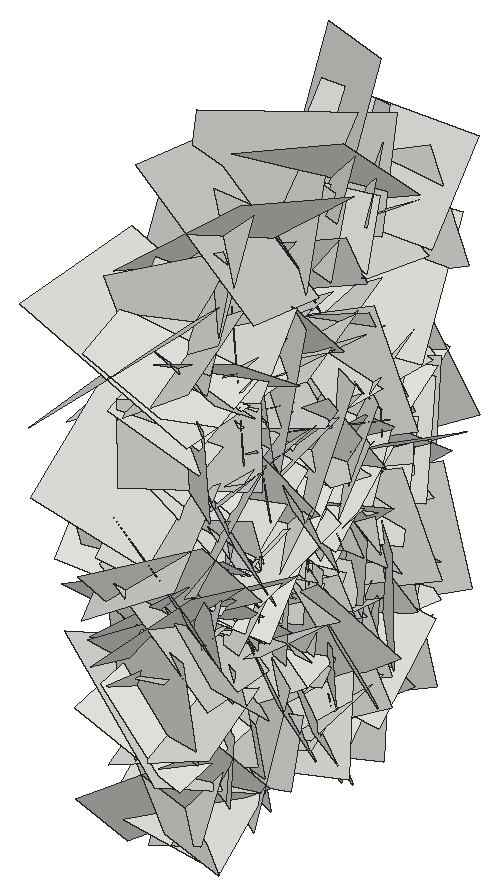
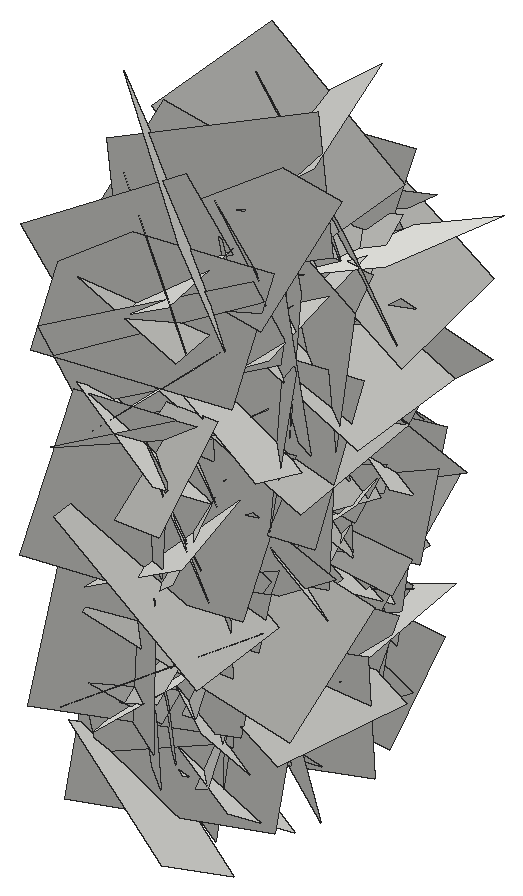
# SketchUp Ruby script. Lengths in inches.
U = 1.inch
M = Sketchup.active_model
def pt(a) = Geom::Point3d.new(a.map { |v| v * U })
def face(e, loops, mat)
  f = e.add_face(loops[0].map { |a| pt(a) })
  loops[1..].each { |l| e.add_face(l.map { |a| pt(a) }).erase! }
  f.material = f.back_material = mat if mat
  f
end
# faces: each face lists its corners as indices into pts; further lists are holes
def faces(e, pts, list, mat = nil) = list.each { |f| face(e, (f[0].is_a?(Array) ? f : [f]).map { |l| l.map { |i| pts[i] } }, mat) }
# xy, xz, yz: faces in a plane at the given z, y or x. An outline is a flat list of corners, or four numbers for a rectangle; further outlines are holes
def ring(l) = l.size == 4 ? [[l[0], l[1]], [l[2], l[1]], [l[2], l[3]], [l[0], l[3]]] : l.each_slice(2).to_a
def flat(e, list, mat, &to3) = list.each { |f| face(e, (f[0].is_a?(Array) ? f : [f]).map { |l| ring(l).map { |u, v| to3.(u, v) } }, mat) }
def xy(e, z, list, mat = nil) = flat(e, list, mat) { |x, y| [x, y, z] }
def xz(e, y, list, mat = nil) = flat(e, list, mat) { |x, z| [x, y, z] }
def yz(e, x, list, mat = nil) = flat(e, list, mat) { |y, z| [x, y, z] }
def lines(e, pts, list) = list.each { |a, b| e.add_line(pt(pts[a]), pt(pts[b])) }
# prism: a flat outline (further loops are holes) pulled along v
def prism(e, loops, v, mat = nil)
  f = face(e, loops, mat); d = Geom::Vector3d.new(v.map { |x| x * U })
  f.pushpull(f.normal.samedirection?(d) ? d.length : -d.length)
end
def box(e, o, s, mat = nil) = prism(e, [[o, [o[0] + s[0], o[1], o[2]], [o[0] + s[0], o[1] + s[1], o[2]], [o[0], o[1] + s[1], o[2]]]], [0, 0, s[2]], mat)
def at(x, y, z, deg = 0) = Geom::Transformation.translation(pt([x, y, z])) * Geom::Transformation.rotation(ORIGIN, Z_AXIS, deg.degrees)
def axes(o, x, y, z) = Geom::Transformation.new([*x, 0, *y, 0, *z, 0, *pt(o).to_a, 1])
def part(name) = M.definitions.add(name)
# library, detail: a bought-in or finely detailed component or shape, given as its bounding box
def library(name, o, s) = part(name).tap { |d| box(d.entities, o, s) }
def detail(e, o, s) = box(e.add_group.entities, o, s)
def put(e, d, t, mat = nil) = e.add_instance(d, t).tap { |i| i.material = mat if mat }
def group(e, t, mat = nil) = e.add_group.tap { |g| g.transformation = t; g.material = mat if mat }.entities
root = M.entities
c1 = part("Component\#6")
p = [[0.01,0,0],[0,3.24,4.54],[4.32,3.24,4.54],[4.33,0,0]]
faces(c1.entities,p,[[0,1,2,3]])
put(root,c1,axes([18.5,148.21,18.05],[-0.18781,1.38239,0.05917],[-0.11095,0.04609,-1.39025],[-1.46247,-0.18102,0.09787]))
put(root,c1,axes([18.5,151.36,16.73],[-0.05564,-1.33407,-0.12972],[-0.26745,-0.11766,1.31218],[-1.39538,0.07575,-0.24633]))
put(root,c1,axes([18.5,153.54,10.59],[-0.17173,1.22834,-0.55665],[-0.01226,-0.5619,-1.23655],[-1.42944,-0.14275,0.07748]))
put(root,c1,axes([18.5,150.02,13.53],[-0.11354,-0.10924,1.28227],[-0.18202,1.27641,0.09439],[-1.35193,-0.16268,-0.1204]))
put(root,c1,axes([18.5,150.46,17.01],[-0.04698,1.34267,-0.16756],[-0.13374,-0.17102,-1.33703],[-1.42802,-0.02815,0.13073]))
put(root,c1,axes([18.5,146.56,18.67],[-0.08115,0.67304,1.19325],[-0.03541,1.19384,-0.67552],[-1.45175,-0.06674,-0.05023]))
put(root,c1,axes([18.5,155.15,17.37],[-0.02517,0.60882,-1.16754],[-0.2041,-1.15679,-0.59929],[-1.38075,0.1599,0.10987]))
put(root,c1,axes([18.5,149.47,1.18],[-0.22795,-1.08393,0.44752],[-0.03192,0.45993,1.09954],[-1.24263,0.18702,-0.11034]))
put(root,c1,axes([18.5,145.22,20.96],[-0.20751,1.35949,-0.09859],[0.20583,-0.07077,-1.36145],[-1.43011,-0.20745,-0.18164]))
put(root,c1,axes([18.5,151.77,16.16],[-0.14743,1.12249,0.38129],[-0.0578,0.37744,-1.13105],[-1.25528,-0.14922,0.00729]))
put(root,c1,axes([18.5,155.16,12.125],[-0.20792,1.23942,0.0793],[0.14973,0.10203,-1.24521],[-1.30793,-0.18535,-0.15516]))
put(root,c1,axes([18.5,149.82,11.51],[-0.16938,-0.10345,1.35904],[0.25816,1.34416,0.13095],[-1.4215,0.25644,-0.13816]))
put(root,c1,axes([18.5,149.27,6.59],[0.15688,1.33929,-0.00269],[-0.18956,0.01708,-1.33541],[-1.40693,0.14704,0.17962]))
put(root,c1,axes([18.5,157.09,9.16],[-0.26081,-0.66319,-0.77037],[-0.09697,-0.77495,0.69635],[-1.07312,0.23121,0.12431]))
put(root,c1,axes([18.5,153.21,11.43],[0.14123,-0.96535,-0.93141],[-0.15435,-0.94087,0.95433],[-1.41351,0.00629,-0.19727]))
put(root,c1,axes([18.5,154.4,5.48],[0.14525,-0.2612,-1.20099],[-0.27145,-1.18798,0.22915],[-1.27422,0.2233,-0.18571]))
put(root,c1,axes([18.5,153.41,21.56],[-0.04666,0.60871,1.19242],[0.17987,1.18598,-0.59916],[-1.40769,0.13136,-0.11609]))
put(root,c1,axes([18.5,152.41,8.09],[0.02535,-1.06677,0.60381],[-0.0625,0.60222,1.06631],[-1.29785,-0.04984,-0.03955]))
put(root,c1,axes([18.5,151.84,12.71],[-0.09641,-0.969,-0.91768],[0.24854,-0.9171,0.94515],[-1.39265,-0.09659,0.2322]))
put(root,c1,axes([18.5,148.37,14.37],[-0.13394,0.02599,1.3483],[0.3112,1.32226,0.00203],[-1.39518,0.29244,-0.12899]))
put(root,c1,axes([18.5,148.8125,12.02],[-0.02959,0.36254,-1.01381],[-0.21176,-0.99828,-0.35148],[-1.12146,0.17893,0.09312]))
put(root,c1,axes([18.5,153.72,24.55],[0.10736,0.8301,-0.78481],[-0.26067,-0.75358,-0.8288],[-1.18252,0.24148,0.11144]))
put(root,c1,axes([18.5,144.59,11.1],[-0.20686,0.83944,0.54314],[-0.00436,0.55271,-0.85571],[-1.05982,-0.16612,-0.10249]))
put(root,c1,axes([18.5,150.33,13.2],[0.24126,0.02501,1.36725],[-0.05252,1.3853,-0.01709],[-1.44858,-0.04606,0.22834]))
put(root,c1,axes([18.5,153.16,13.74],[-0.07693,-1.07175,0.44962],[0.07215,0.4458,1.07364],[-1.22986,0.09319,0.03486]))
put(root,c1,axes([14.53,155.94,6.59],[-0.14653,0.65267,0.04592],[-0.0729,0.03218,-0.6644],[0.6897,0.14207,-0.06047]))
put(root,c1,axes([18.5,147.25,11.15],[-0.01251,0.83252,-0.66438],[-0.16644,-0.65852,-0.82239],[-1.1167,0.08883,0.13002]))
put(root,c1,axes([18.5,157.5,5.99],[-0.02733,0.34478,-1.12821],[0.04378,-1.12752,-0.34552],[-1.24973,-0.04704,0.01257]))
put(root,c1,axes([18.5,159.05,4.5],[-0.22831,-0.97739,-0.02602],[0.01319,-0.02938,1.00067],[-1.03632,0.21495,0.01847]))
put(root,c1,axes([18.5,156.09,10.89],[-0.02844,-1.01096,-0.23497],[-0.17327,-0.228,0.99963],[-1.08645,0.06282,-0.15327]))
put(root,c1,axes([18.5,158.38,15.93],[0.03304,0.59909,-1.16183],[0.1621,-1.15585,-0.5919],[-1.37611,-0.12177,-0.09762]))
put(root,c1,axes([18.5,147.43,1.76],[-0.0449,0.15818,1.07958],[-0.0304,1.07985,-0.15935],[-1.15617,-0.03454,-0.03773]))
put(root,c1,axes([18.5,156.6875,24.44],[-0.16473,0.01802,-1.18121],[0.23771,-1.16927,-0.04735],[-1.22945,-0.22849,0.14911]))
put(root,c1,axes([14.53,148.65,3.04],[-0.12439,-0.47488,0.46679],[-0.05284,0.47892,0.47469],[0.70386,-0.04797,0.11813]))
put(root,c1,axes([14.53,150.18,6.375],[-0.17639,-0.58204,-0.33942],[0.00316,-0.35025,0.59915],[0.71419,-0.1422,-0.08648]))
put(root,c1,axes([18.5,151.75,19.45],[-0.16935,0.44212,0.83371],[-0.05466,0.84022,-0.45546],[-0.99881,-0.12095,-0.11643]))
put(root,c1,axes([18.5,152.08,1.74],[-0.04493,0.85391,0.54577],[-0.09586,0.54089,-0.85328],[-1.06994,-0.08432,0.05353]))
put(root,c1,axes([18.5,158.83,13.98],[-0.00743,-1.2386,0.03478],[0.17851,0.0335,1.22715],[-1.30124,0.01167,0.16814]))
put(root,c1,axes([18.5,148.93,-0.125],[0.17085,0.2332,1.25619],[0.02467,1.2654,-0.2379],[-1.35409,0.05247,0.15416]))
put(root,c1,axes([18.5,148.09,7.11],[0.15706,0.67864,1.02073],[-0.03183,1.02986,-0.68036],[-1.29889,0.05683,0.1401]))
put(root,c1,axes([18.5,145.87,3.84],[-0.08046,-0.07863,0.91675],[-0.19442,0.90269,0.06223],[-0.95574,-0.17701,-0.08983]))
put(root,c1,axes([18.5,155.4,17.52],[0.19723,0.3027,-1.19403],[-0.0763,-1.20284,-0.31615],[-1.30348,0.11621,-0.16216]))
put(root,c1,axes([18.5,148.31,17.26],[-0.09379,0.98835,0.28145],[0.01751,0.28383,-0.99149],[-1.08916,-0.08054,-0.04018]))
put(root,c1,axes([18.5,151.01,19.39],[-0.01021,0.65154,-0.69294],[-0.23408,-0.67557,-0.63214],[-0.98066,0.15447,0.1581]))
put(root,c1,axes([18.5,157.43,12.97],[0.1074,-0.05602,-1.35571],[0.22854,-1.34155,0.07155],[-1.42001,-0.22014,-0.09102]))
put(root,c1,axes([14.53,152.72,13.34],[-0.14332,-0.62648,-0.12325],[0.10799,-0.14554,0.62801],[0.66813,-0.11086,-0.12794]))
put(root,c1,axes([18.5,154.9,1.8],[-0.03269,0.90387,0.50014],[-0.00572,0.50021,-0.90434],[-1.09498,-0.0296,-0.01021]))
put(root,c1,axes([14.53,149.02,5.32],[-0.19432,-0.67994,0.40742],[-0.04988,0.42677,0.69106],[0.83874,-0.13215,0.13549]))
put(root,c1,axes([18.5,160.22,19.0625],[0.13961,-0.68099,-1.03193],[0.07146,-1.03227,0.68982],[-1.30861,-0.12902,-0.07242]))
put(root,c1,axes([18.5,157.74,11.21],[-0.0595,-0.6331,0.72554],[-0.06262,0.72766,0.63038],[-1.01877,-0.00775,-0.08112]))
put(root,c1,axes([14.53,146,16.15],[-0.10062,0.63244,0.10884],[0.07256,0.11937,-0.63396],[0.67636,0.08128,0.0842]))
put(root,c1,axes([14.53,147.25,18.09],[-0.11506,-0.20062,0.68841],[-0.02156,0.69683,0.19986],[0.75976,-0.01061,0.10993]))
put(root,c1,axes([14.53,155.37,8.05],[-0.03179,-0.04018,0.69029],[-0.07893,0.6871,0.03676],[0.72868,0.07267,0.03409]))
put(root,c1,axes([14.53,151.91,13.09],[-0.06029,-0.61389,0.14039],[0.0496,0.13645,0.61563],[0.66568,-0.06576,-0.03315]))
put(root,c1,axes([18.5,153.47,7.93],[0.25077,0.36385,-1.26635],[0.08689,-1.28818,-0.35481],[-1.39394,-0.01484,-0.24993]))
put(root,c1,axes([18.5,158.45,22.43],[0.19892,0.24365,-1.12098],[-0.08242,-1.13056,-0.25875],[-1.21318,0.11676,-0.16622]))
put(root,c1,axes([14.53,151.13,9.12],[-0.15296,0.67587,0.31221],[0.03502,0.32352,-0.68509],[0.78839,0.11676,0.09101]))
put(root,c1,axes([18.5,148.76,4.0625],[-0.10183,-0.75916,-0.2873],[-0.20096,-0.26032,0.75126],[-0.83661,0.15493,-0.14549]))
put(root,c1,axes([18.5,155.05,20.66],[-0.11898,0.43702,0.87755],[0.10329,0.88388,-0.42771],[-1.03402,0.038,-0.1437]))
put(root,c1,axes([18.5,154.79,8.7],[0.06507,0.61236,-0.89404],[0.03144,-0.89608,-0.61173],[-1.14823,0.01016,-0.06741]))
put(root,c1,axes([14.53,151.99,2.12],[-0.1775,0.68354,0.35821],[0.06031,0.37649,-0.69181],[0.81579,0.12089,0.12909]))
put(root,c1,axes([14.53,151.79,4.27],[-0.00282,-0.67031,0.14172],[-0.04158,0.14164,0.66918],[0.72504,0.00552,0.03892]))
put(root,c1,axes([14.53,147.62,1.41],[-0.08717,-0.06025,0.7019],[0.04865,0.70471,0.06586],[0.74517,-0.05306,0.07781]))
put(root,c1,axes([14.53,156.87,7.65],[0.00449,0.50233,-0.39291],[0.02578,-0.39276,-0.50188],[0.67552,0.01165,0.02176]))
put(root,c1,axes([14.53,153.92,20.8125],[0.01755,0.277,-0.54123],[0.05617,-0.54003,-0.27476],[0.64202,0.03967,0.03883]))
put(root,c1,axes([18.5,152.6,3.91],[-0.02426,0.68313,0.69515],[0.0107,0.69547,-0.68312],[-1.03305,-0.00884,-0.0234]))
put(root,c1,axes([14.53,147.13,6.96],[-0.04816,-0.19283,0.63159],[0.07038,0.62854,0.19668],[0.69645,-0.07685,0.0238]))
put(root,c1,axes([18.5,158.68,8.63],[0.07829,-0.94373,0.27717],[-0.10215,0.26967,0.94388],[-1.03759,-0.09775,-0.07202]))
put(root,c1,axes([18.5,152.91,14.99],[0.05042,0.65822,-0.8803],[0.11398,-0.87969,-0.65195],[-1.15954,-0.05785,-0.10236]))
put(root,c1,axes([18.5,159.16,9.85],[0.13765,0.1916,-1.18129],[0.14512,-1.1828,-0.17679],[-1.2602,-0.11528,-0.14939]))
put(root,c1,axes([18.5,157.06,14.03],[0.04606,-0.47436,-0.98882],[0.12961,-0.98133,0.47614],[-1.15527,-0.12901,0.01399]))
put(root,c1,axes([18.5,149.64,15.49],[0.05397,-0.71515,0.49033],[-0.26351,0.45852,0.69456],[-0.88054,-0.18105,-0.1778]))
put(root,c1,axes([14.53,148.39,13.69],[0.056,0.56116,0.2115],[0.06403,0.20626,-0.56234],[0.63244,-0.07057,0.03821]))
put(root,c1,axes([18.5,147.71,9.53],[0.0202,0.73421,-0.62443],[-0.01239,-0.62433,-0.73445],[-1.02159,0.02209,-0.00344]))
put(root,c1,axes([14.53,146.72,8.375],[0.05548,0.31048,0.67068],[-0.12303,0.66747,-0.29994],[0.77368,0.08387,-0.09579]))
put(root,c1,axes([18.5,152.28,1.18],[0.22482,-0.75958,0.923],[0.06114,0.94282,0.76264],[-1.2656,-0.08938,0.2008]))
put(root,c1,axes([18.5,154.73,4.99],[0.23466,-0.21907,1.02966],[-0.17179,1.03255,0.25453],[-1.10257,-0.20751,0.17949]))
put(root,c1,axes([14.53,148.44,10.1],[0.02371,0.59128,0.15103],[0.13632,0.14317,-0.57956],[0.63236,-0.05303,0.11928]))
put(root,c1,axes([14.53,154.81,5.31],[0.03271,-0.68931,-0.29186],[-0.0897,-0.29345,0.68411],[0.78838,-0.00479,0.08995]))
put(root,c1,axes([14.53,155.07,5.6],[-0.26442,-0.95782,0.42161],[-0.12666,0.45666,0.96674],[1.10204,-0.17733,0.21227]))
put(root,c1,axes([18.5,146.38,17.95],[-0.09245,0.38694,0.78979],[0.04684,0.79459,-0.38441],[-0.93107,0.00155,-0.09776]))
put(root,c1,axes([14.53,155.43,2.74],[0.05213,0.12024,0.7107],[-0.06472,0.71048,-0.11598],[0.7613,0.05216,-0.05853]))
put(root,c1,axes([18.5,149.03,14.67],[0.12882,0.64149,-0.81464],[-0.00451,-0.8199,-0.64626],[-1.09909,0.07855,-0.09282]))
put(root,c1,axes([14.53,145.53,10.42],[-0.22479,1.04725,-0.16356],[-0.16331,-0.19548,-1.05191],[1.11161,0.18306,-0.18761]))
put(root,c1,axes([18.5,147.21,13.43],[0.06341,1.09172,0.23851],[0.19798,0.22572,-1.08003],[-1.16785,0.09755,-0.17015]))
put(root,c1,axes([14.53,146.09,12.1875],[-0.18427,0.52878,-0.65011],[0.11203,-0.64482,-0.55274],[0.8812,0.19255,-0.06567]))
put(root,c1,axes([18.5,151.57,3.27],[-0.14157,0.02397,-0.74069],[-0.04702,-0.75154,-0.01632],[-0.78414,0.04073,0.1347]))
put(root,c1,axes([14.53,154.48,3.89],[0.11783,0.23417,0.69133],[-0.11259,0.69704,-0.21902],[0.76547,0.06648,-0.13863]))
put(root,c1,axes([14.53,152.53,7.1875],[0.08757,-0.64703,0.3684],[-0.09594,0.35919,0.65114],[0.78338,0.11632,0.03856]))
put(root,c1,axes([18.5,153.68,-0.24],[-0.08313,-0.05331,0.78078],[-0.05564,0.78328,0.04821],[-0.82769,-0.0473,-0.08166]))
put(root,c1,axes([14.53,155.23,10.47],[-0.04155,0.12694,-0.87349],[-0.11983,-0.86787,-0.12105],[0.92792,-0.10639,-0.05475]))
put(root,c1,axes([18.5,154.93,13.48],[0.13332,0.92748,-0.67904],[0.1887,-0.69057,-0.91025],[-1.20375,-0.00553,-0.2179]))
put(root,c1,axes([18.5,152.46,19.1],[0.24316,-1.11668,0.32256],[0.08367,0.34299,1.13127],[-1.22923,-0.19755,0.14081]))
put(root,c1,axes([18.5,149.625,17.57],[-0.05592,-0.7816,-0.40589],[0.0657,-0.4089,0.77935],[-0.93124,0.01809,0.07936]))
put(root,c1,axes([14.53,153.02,6.56],[0.04835,0.51462,-0.41299],[0.10228,-0.41473,-0.50612],[0.69191,0.02534,0.10368]))
put(root,c1,axes([14.53,155.74,21.65],[-0.00825,-0.17983,-0.66547],[0.14401,-0.65286,0.17483],[0.71636,0.12918,-0.04281]))
put(root,c1,axes([18.5,147.06,-0.97],[-0.01135,-0.66277,0.66685],[0.09721,0.66298,0.66039],[-0.99185,0.07256,0.05709]))
put(root,c1,axes([14.53,154.86,6.54],[-0.11481,0.21277,-0.79232],[0.09254,-0.79167,-0.22453],[0.86468,0.11298,-0.08117]))
put(root,c1,axes([18.5,155.95,10.68],[-0.04823,-0.00518,0.84226],[0.02844,0.84305,0.00663],[-0.89236,0.02715,-0.04531]))
put(root,c1,axes([18.5,146.53,12.92],[-0.03124,-0.05121,0.8385],[0.00373,0.839,0.05136],[-0.89046,0.00531,-0.0292]))
put(root,c1,axes([18.5,152.8,10.75],[0.04843,-0.82009,-0.82841],[0.32646,-0.79109,0.80013],[-1.19171,-0.25004,0.18553]))
put(root,c1,axes([14.53,155.82,10.86],[-0.10869,-0.77244,0.23734],[0.13092,0.22145,0.77409],[0.8465,-0.13343,-0.08925]))
put(root,c1,axes([14.53,156.49,11.61],[-0.16435,-0.92659,-0.48849],[-0.14398,-0.47186,0.93815],[1.10094,-0.20004,0.04977]))
put(root,c1,axes([18.5,153.88,7.81],[-0.12498,-0.19712,-0.75186],[0.05107,-0.76085,0.19192],[-0.82232,-0.01729,0.12619]))
put(root,c1,axes([14.53,154.72,7.86],[0.01434,-0.12328,-0.7123],[0.10241,-0.70572,0.12398],[0.75939,0.0975,-0.00327]))
put(root,c1,axes([18.5,155.22,14.18],[0.0107,0.67836,0.43703],[-0.08223,0.43585,-0.67474],[-0.8514,-0.03357,0.07066]))
put(root,c1,axes([14.53,152.55,8.85],[-0.17208,0.39932,0.93109],[-0.08126,0.93542,-0.41455],[1.07081,0.13515,0.11817]))
put(root,c1,axes([18.5,155.14,21.07],[0.01676,0.7943,-0.14622],[-0.08914,-0.14383,-0.79043],[-0.85145,0.03069,0.07988]))
put(root,c1,axes([14.53,158.76,13.54],[-0.17018,-0.33172,-0.9968],[-0.1229,-0.99662,0.35033],[1.10678,-0.16167,-0.11436]))
put(root,c1,axes([18.5,151.77,10.3],[-0.00621,-0.04081,-0.81439],[-0.02737,-0.814,0.04098],[-0.86391,0.02608,0.00455]))
put(root,c1,axes([18.5,149.67,1.32],[-0.10197,-0.47157,-0.58691],[0.00963,-0.59236,0.47447],[-0.798,0.05311,0.08072]))
put(root,c1,axes([14.53,154.27,5.56],[-0.10843,0.64197,-0.78685],[-0.13439,-0.79271,-0.63027],[1.06801,-0.03458,-0.15919]))
put(root,c1,axes([18.5,154.27,5.56],[0.10843,0.64197,-0.78685],[0.13439,-0.79271,-0.63027],[-1.06801,-0.03458,-0.15919]))
put(root,c1,axes([14.53,149.67,1.32],[0.10197,-0.47157,-0.58691],[-0.00963,-0.59236,0.47447],[0.798,0.05311,0.08072]))
put(root,c1,axes([14.53,151.77,10.3],[0.00621,-0.04081,-0.81439],[0.02737,-0.814,0.04098],[0.86391,0.02608,0.00455]))
put(root,c1,axes([18.5,158.76,13.54],[0.17018,-0.33172,-0.9968],[0.1229,-0.99662,0.35033],[-1.10678,-0.16167,-0.11436]))
put(root,c1,axes([14.53,155.14,21.07],[-0.01676,0.7943,-0.14622],[0.08914,-0.14383,-0.79043],[0.85145,0.03069,0.07988]))
put(root,c1,axes([18.5,152.55,8.85],[0.17208,0.39932,0.93109],[0.08126,0.93542,-0.41455],[-1.07081,0.13515,0.11817]))
put(root,c1,axes([14.53,155.22,14.18],[-0.0107,0.67836,0.43703],[0.08223,0.43585,-0.67474],[0.8514,-0.03357,0.07066]))
put(root,c1,axes([18.5,154.72,7.86],[-0.01434,-0.12328,-0.7123],[-0.10241,-0.70572,0.12398],[-0.75939,0.0975,-0.00327]))
put(root,c1,axes([14.53,153.88,7.81],[0.12498,-0.19712,-0.75186],[-0.05107,-0.76085,0.19192],[0.82232,-0.01729,0.12619]))
put(root,c1,axes([18.5,156.49,11.61],[0.16435,-0.92659,-0.48849],[0.14398,-0.47186,0.93815],[-1.10094,-0.20004,0.04977]))
put(root,c1,axes([18.5,155.82,10.86],[0.10869,-0.77244,0.23734],[-0.13092,0.22145,0.77409],[-0.8465,-0.13343,-0.08925]))
put(root,c1,axes([14.53,152.8,10.75],[-0.04843,-0.82009,-0.82841],[-0.32646,-0.79109,0.80013],[1.19171,-0.25004,0.18553]))
put(root,c1,axes([14.53,146.53,12.92],[0.03124,-0.05121,0.8385],[-0.00373,0.839,0.05136],[0.89046,0.00531,-0.0292]))
put(root,c1,axes([14.53,155.95,10.68],[0.04823,-0.00518,0.84226],[-0.02844,0.84305,0.00663],[0.89236,0.02715,-0.04531]))
put(root,c1,axes([18.5,154.86,6.54],[0.11481,0.21277,-0.79232],[-0.09254,-0.79167,-0.22453],[-0.86468,0.11298,-0.08117]))
put(root,c1,axes([14.53,147.06,-0.97],[0.01135,-0.66277,0.66685],[-0.09721,0.66298,0.66039],[0.99185,0.07256,0.05709]))
put(root,c1,axes([18.5,155.74,21.65],[0.00825,-0.17983,-0.66547],[-0.14401,-0.65286,0.17483],[-0.71636,0.12918,-0.04281]))
put(root,c1,axes([18.5,153.02,6.56],[-0.04835,0.51462,-0.41299],[-0.10228,-0.41473,-0.50612],[-0.69191,0.02534,0.10368]))
put(root,c1,axes([14.53,149.625,17.57],[0.05592,-0.7816,-0.40589],[-0.0657,-0.4089,0.77935],[0.93124,0.01809,0.07936]))
put(root,c1,axes([14.53,152.46,19.1],[-0.24316,-1.11668,0.32256],[-0.08367,0.34299,1.13127],[1.22923,-0.19755,0.14081]))
put(root,c1,axes([14.53,154.93,13.48],[-0.13332,0.92748,-0.67904],[-0.1887,-0.69057,-0.91025],[1.20375,-0.00553,-0.2179]))
put(root,c1,axes([18.5,155.23,10.47],[0.04155,0.12694,-0.87349],[0.11983,-0.86787,-0.12105],[-0.92792,-0.10639,-0.05475]))
put(root,c1,axes([14.53,153.68,-0.24],[0.08313,-0.05331,0.78078],[0.05564,0.78328,0.04821],[0.82769,-0.0473,-0.08166]))
put(root,c1,axes([18.5,152.53,7.1875],[-0.08757,-0.64703,0.3684],[0.09594,0.35919,0.65114],[-0.78338,0.11632,0.03856]))
put(root,c1,axes([18.5,154.48,3.89],[-0.11783,0.23417,0.69133],[0.11259,0.69704,-0.21902],[-0.76547,0.06648,-0.13863]))
put(root,c1,axes([14.53,151.57,3.27],[0.14157,0.02397,-0.74069],[0.04702,-0.75154,-0.01632],[0.78414,0.04073,0.1347]))
put(root,c1,axes([18.5,146.09,12.1875],[0.18427,0.52878,-0.65011],[-0.11203,-0.64482,-0.55274],[-0.8812,0.19255,-0.06567]))
put(root,c1,axes([14.53,147.21,13.43],[-0.06341,1.09172,0.23851],[-0.19798,0.22572,-1.08003],[1.16785,0.09755,-0.17015]))
put(root,c1,axes([18.5,145.53,10.42],[0.22479,1.04725,-0.16356],[0.16331,-0.19548,-1.05191],[-1.11161,0.18306,-0.18761]))
put(root,c1,axes([14.53,149.03,14.67],[-0.12882,0.64149,-0.81464],[0.00451,-0.8199,-0.64626],[1.09909,0.07855,-0.09282]))
put(root,c1,axes([18.5,155.43,2.74],[-0.05213,0.12024,0.7107],[0.06472,0.71048,-0.11598],[-0.7613,0.05216,-0.05853]))
put(root,c1,axes([14.53,146.38,17.95],[0.09245,0.38694,0.78979],[-0.04684,0.79459,-0.38441],[0.93107,0.00155,-0.09776]))
put(root,c1,axes([18.5,155.07,5.6],[0.26442,-0.95782,0.42161],[0.12666,0.45666,0.96674],[-1.10204,-0.17733,0.21227]))
put(root,c1,axes([18.5,154.81,5.31],[-0.03271,-0.68931,-0.29186],[0.0897,-0.29345,0.68411],[-0.78838,-0.00479,0.08995]))
put(root,c1,axes([18.5,148.44,10.1],[-0.02371,0.59128,0.15103],[-0.13632,0.14317,-0.57956],[-0.63236,-0.05303,0.11928]))
put(root,c1,axes([14.53,154.73,4.99],[-0.23466,-0.21907,1.02966],[0.17179,1.03255,0.25453],[1.10257,-0.20751,0.17949]))
put(root,c1,axes([14.53,152.28,1.18],[-0.22482,-0.75958,0.923],[-0.06114,0.94282,0.76264],[1.2656,-0.08938,0.2008]))
put(root,c1,axes([18.5,146.72,8.375],[-0.05548,0.31048,0.67068],[0.12303,0.66747,-0.29994],[-0.77368,0.08387,-0.09579]))
put(root,c1,axes([14.53,147.71,9.53],[-0.0202,0.73421,-0.62443],[0.01239,-0.62433,-0.73445],[1.02159,0.02209,-0.00344]))
put(root,c1,axes([18.5,148.39,13.69],[-0.056,0.56116,0.2115],[-0.06403,0.20626,-0.56234],[-0.63244,-0.07057,0.03821]))
put(root,c1,axes([14.53,149.64,15.49],[-0.05397,-0.71515,0.49033],[0.26351,0.45852,0.69456],[0.88054,-0.18105,-0.1778]))
put(root,c1,axes([14.53,157.06,14.03],[-0.04606,-0.47436,-0.98882],[-0.12961,-0.98133,0.47614],[1.15527,-0.12901,0.01399]))
put(root,c1,axes([14.53,159.16,9.85],[-0.13765,0.1916,-1.18129],[-0.14512,-1.1828,-0.17679],[1.2602,-0.11528,-0.14939]))
put(root,c1,axes([14.53,152.91,14.99],[-0.05042,0.65822,-0.8803],[-0.11398,-0.87969,-0.65195],[1.15954,-0.05785,-0.10236]))
put(root,c1,axes([14.53,158.68,8.63],[-0.07829,-0.94373,0.27717],[0.10215,0.26967,0.94388],[1.03759,-0.09775,-0.07202]))
put(root,c1,axes([18.5,147.13,6.96],[0.04816,-0.19283,0.63159],[-0.07038,0.62854,0.19668],[-0.69645,-0.07685,0.0238]))
put(root,c1,axes([14.53,152.6,3.91],[0.02426,0.68313,0.69515],[-0.0107,0.69547,-0.68312],[1.03305,-0.00884,-0.0234]))
put(root,c1,axes([18.5,153.92,20.8125],[-0.01755,0.277,-0.54123],[-0.05617,-0.54003,-0.27476],[-0.64202,0.03967,0.03883]))
put(root,c1,axes([18.5,156.87,7.65],[-0.00449,0.50233,-0.39291],[-0.02578,-0.39276,-0.50188],[-0.67552,0.01165,0.02176]))
put(root,c1,axes([18.5,147.62,1.41],[0.08717,-0.06025,0.7019],[-0.04865,0.70471,0.06586],[-0.74517,-0.05306,0.07781]))
put(root,c1,axes([18.5,151.79,4.27],[0.00282,-0.67031,0.14172],[0.04158,0.14164,0.66918],[-0.72504,0.00552,0.03892]))
put(root,c1,axes([18.5,151.99,2.12],[0.1775,0.68354,0.35821],[-0.06031,0.37649,-0.69181],[-0.81579,0.12089,0.12909]))
put(root,c1,axes([14.53,154.79,8.7],[-0.06507,0.61236,-0.89404],[-0.03144,-0.89608,-0.61173],[1.14823,0.01016,-0.06741]))
put(root,c1,axes([14.53,155.05,20.66],[0.11898,0.43702,0.87755],[-0.10329,0.88388,-0.42771],[1.03402,0.038,-0.1437]))
put(root,c1,axes([14.53,148.76,4.0625],[0.10183,-0.75916,-0.2873],[0.20096,-0.26032,0.75126],[0.83661,0.15493,-0.14549]))
put(root,c1,axes([18.5,151.13,9.12],[0.15296,0.67587,0.31221],[-0.03502,0.32352,-0.68509],[-0.78839,0.11676,0.09101]))
